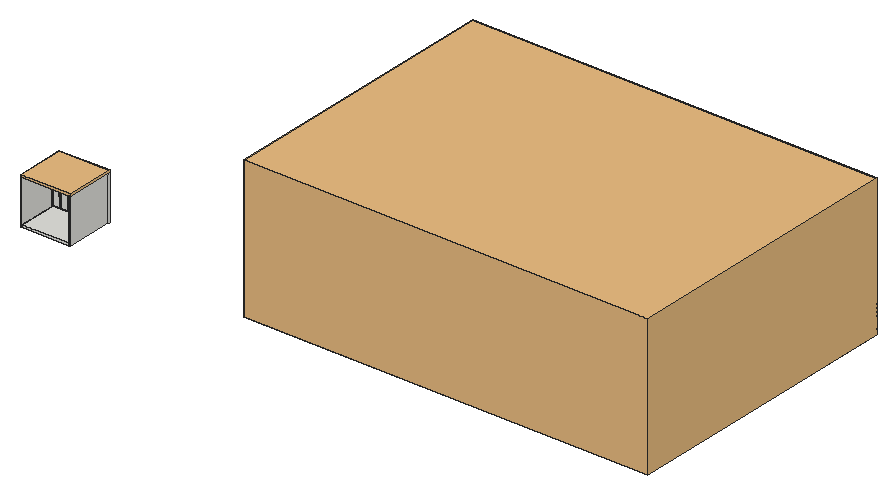
# SketchUp Ruby script. Lengths in inches.
U = 1.inch
M = Sketchup.active_model
def pt(a) = Geom::Point3d.new(a.map { |v| v * U })
def face(e, loops, mat)
  f = e.add_face(loops[0].map { |a| pt(a) })
  loops[1..].each { |l| e.add_face(l.map { |a| pt(a) }).erase! }
  f.material = f.back_material = mat if mat
  f
end
# faces: each face lists its corners as indices into pts; further lists are holes
def faces(e, pts, list, mat = nil) = list.each { |f| face(e, (f[0].is_a?(Array) ? f : [f]).map { |l| l.map { |i| pts[i] } }, mat) }
# xy, xz, yz: faces in a plane at the given z, y or x. An outline is a flat list of corners, or four numbers for a rectangle; further outlines are holes
def ring(l) = l.size == 4 ? [[l[0], l[1]], [l[2], l[1]], [l[2], l[3]], [l[0], l[3]]] : l.each_slice(2).to_a
def flat(e, list, mat, &to3) = list.each { |f| face(e, (f[0].is_a?(Array) ? f : [f]).map { |l| ring(l).map { |u, v| to3.(u, v) } }, mat) }
def xy(e, z, list, mat = nil) = flat(e, list, mat) { |x, y| [x, y, z] }
def xz(e, y, list, mat = nil) = flat(e, list, mat) { |x, z| [x, y, z] }
def yz(e, x, list, mat = nil) = flat(e, list, mat) { |y, z| [x, y, z] }
def lines(e, pts, list) = list.each { |a, b| e.add_line(pt(pts[a]), pt(pts[b])) }
# prism: a flat outline (further loops are holes) pulled along v
def prism(e, loops, v, mat = nil)
  f = face(e, loops, mat); d = Geom::Vector3d.new(v.map { |x| x * U })
  f.pushpull(f.normal.samedirection?(d) ? d.length : -d.length)
end
def box(e, o, s, mat = nil) = prism(e, [[o, [o[0] + s[0], o[1], o[2]], [o[0] + s[0], o[1] + s[1], o[2]], [o[0], o[1] + s[1], o[2]]]], [0, 0, s[2]], mat)
def at(x, y, z, deg = 0) = Geom::Transformation.translation(pt([x, y, z])) * Geom::Transformation.rotation(ORIGIN, Z_AXIS, deg.degrees)
def axes(o, x, y, z) = Geom::Transformation.new([*x, 0, *y, 0, *z, 0, *pt(o).to_a, 1])
def part(name) = M.definitions.add(name)
# library, detail: a bought-in or finely detailed component or shape, given as its bounding box
def library(name, o, s) = part(name).tap { |d| box(d.entities, o, s) }
def detail(e, o, s) = box(e.add_group.entities, o, s)
def put(e, d, t, mat = nil) = e.add_instance(d, t).tap { |i| i.material = mat if mat }
def group(e, t, mat = nil) = e.add_group.tap { |g| g.transformation = t; g.material = mat if mat }.entities
root = M.entities
M.materials.add("[Color A08]").color = [102, 0, 0]
M.materials.add("[Color M09]1").color = [0, 0, 0]
M.materials.add("[Translucent Glass Gray]1").color = [128, 128, 128]
c1 = library("Group\#158",[0,0,0],[1037.25,734.875,359.43])
c2 = part("Group299\#1")
p = [[0,0,0],[0,0,-12.87],[-0.08,0,-12.87],[0.5,-41.15,0],[-0.5,-41.15,0],[0.5,41.15,0],
  [0.5,0,0],[-0.5,41.15,0],[0.08,0,-12.87],[-0.5,0,0],[0,0,-20.82]]
lines(c2.entities,p,[[0,1],[1,2],[3,4],[5,6],[7,5],[1,8],[9,0],[0,6],[8,10],[4,9],[6,3],[2,10],
  [9,7]])
c3 = part("Rectangle Light\#5")
put(c3.entities,c2,at(0,0,0))
c4 = part("Group301\#1")
p = [[0,0,0],[0,0,-12.87],[-0.08,0,-12.87],[0.5,-41.15,0],[-0.5,-41.15,0],[0.5,41.15,0],
  [0.5,0,0],[-0.5,41.15,0],[0.08,0,-12.87],[-0.5,0,0],[0,0,-20.82]]
lines(c4.entities,p,[[0,1],[1,2],[3,4],[5,6],[7,5],[1,8],[9,0],[0,6],[8,10],[4,9],[6,3],[2,10],
  [9,7]])
c5 = part("Rectangle Light\#6")
put(c5.entities,c4,at(0,0,0))
c6 = part("Group\#164")
xy(c6.entities,0,[[1,1,2,2]])
xy(c6.entities,29.73,[[0,1,0.01,1.15,0.06,1.28,0.125,1.375,0.22,1.44,0.35,1.49,0.5,1.5,1,1.5,1,2,0,2]])
xy(c6.entities,48,[[0,1,2,1,2,2,1.15,2,1.15,1.5,0.5,1.5,0.35,1.49,0.22,1.44,0.125,1.375,0.06,1.28,0.01,1.15],[1.11,1.5,1.15,2]])
xz(c6.entities,1,[[1,0,2,0,2,48,0,48,0,29.73,0.14,29.26,0.27,28.79,0.39,28.32,0.5,27.85,0.6,27.375,0.68,26.9,0.76,26.42,0.83,25.9375,0.89,25.45,0.9375,24.97,0.97,24.49,1,24]])
xz(c6.entities,1.5,[[0.5,29.73,0.5,48,1.15,48,1.11,48,1.07,47.98,1.04,47.96,1.02,47.93,1,47.89,1,29.73]])
xz(c6.entities,2,[[1,0,1,24,0.97,24.49,0.9375,24.97,0.89,25.45,0.83,25.9375,0.76,26.42,0.68,26.9,0.6,27.375,0.5,27.85,0.39,28.32,0.27,28.79,0.14,29.26,0,29.73,1,29.73,1,47.89,1.02,47.93,1.04,47.96,1.07,47.98,1.11,48,2,48,2,0]])
yz(c6.entities,1,[[1,0,1.5,24],[1.5,0,2,24],[1.5,29.73,2,47.85],[1.5,47.85,2,47.89]])
yz(c6.entities,2,[[1,0,2,48]])
p = [[0.97,1,24.49],[0.97,1.5,24.49],[1,1.5,24],[1,1,24],[1,2,24],[0.97,2,24.49],
  [0.9375,1,24.97],[0.9375,1.5,24.97],[0.9375,2,24.97],[0.89,1,25.45],[0.89,1.5,25.45],[0.89,2,25.45],
  [0.83,1,25.9375],[0.83,1.5,25.9375],[0.83,2,25.9375],[0.76,1,26.42],[0.76,1.5,26.42],[0.76,2,26.42],
  [0.68,1,26.9],[0.68,1.5,26.9],[0.68,2,26.9],[0.6,1,27.375],[0.6,1.5,27.375],[0.6,2,27.375],
  [0.5,1,27.85],[0.5,1.5,27.85],[0.5,2,27.85],[0.39,1,28.32],[0.39,1.5,28.32],[0.39,2,28.32],
  [0.27,1,28.79],[0.27,1.5,28.79],[0.27,2,28.79],[0.14,1,29.26],[0.14,1.5,29.26],[0.14,2,29.26],
  [0,1,29.73],[0,1.5,29.73],[0,2,29.73],[0,1,48],[0.01,1.15,48],[0.01,1.15,29.73],
  [0.06,1.28,48],[0.06,1.28,29.73],[0.125,1.375,48],[0.125,1.375,29.73],[0.22,1.44,48],[0.22,1.44,29.73],
  [0.35,1.49,48],[0.35,1.49,29.73],[0.5,1.5,48],[0.5,1.5,29.73],[1,2,47.89],[1,1.5,47.89],
  [1.02,1.5,47.93],[1.02,2,47.93],[1.04,1.5,47.96],[1.04,2,47.96],[1.07,1.5,47.98],[1.07,2,47.98],
  [1.11,1.5,48],[1.11,2,48]]
faces(c6.entities,p,[[0,1,2,3],[4,2,1,5],[6,7,1,0],[5,1,7,8],[9,10,7,6],[8,7,10,11],[12,13,10,9],[11,10,13,14],
  [15,16,13,12],[14,13,16,17],[18,19,16,15],[17,16,19,20],[21,22,19,18],[20,19,22,23],[24,25,22,21],[23,22,25,26],
  [27,28,25,24],[26,25,28,29],[30,31,28,27],[29,28,31,32],[33,34,31,30],[32,31,34,35],[36,37,34,33],[35,34,37,38],
  [36,39,40,41],[41,40,42,43],[43,42,44,45],[45,44,46,47],[47,46,48,49],[49,48,50,51],[52,53,54,55],[55,54,56,57],
  [57,56,58,59],[59,58,60,61]])
c7 = part("Group\#163")
xy(c7.entities,0,[[1,1,2,2]])
xy(c7.entities,29.73,[[0,1,0.01,1.15,0.06,1.28,0.125,1.375,0.22,1.44,0.35,1.49,0.5,1.5,1,1.5,1,2,0,2]])
xy(c7.entities,48,[[0,1,2,1,2,2,1.15,2,1.15,1.5,0.5,1.5,0.35,1.49,0.22,1.44,0.125,1.375,0.06,1.28,0.01,1.15],[1.11,1.5,1.15,2]])
xz(c7.entities,1,[[1,0,2,0,2,48,0,48,0,29.73,0.14,29.26,0.27,28.79,0.39,28.32,0.5,27.85,0.6,27.375,0.68,26.9,0.76,26.42,0.83,25.9375,0.89,25.45,0.9375,24.97,0.97,24.49,1,24]])
xz(c7.entities,1.5,[[0.5,29.73,0.5,48,1.15,48,1.11,48,1.07,47.98,1.04,47.96,1.02,47.93,1,47.89,1,29.73]])
xz(c7.entities,2,[[1,0,1,24,0.97,24.49,0.9375,24.97,0.89,25.45,0.83,25.9375,0.76,26.42,0.68,26.9,0.6,27.375,0.5,27.85,0.39,28.32,0.27,28.79,0.14,29.26,0,29.73,1,29.73,1,47.89,1.02,47.93,1.04,47.96,1.07,47.98,1.11,48,2,48,2,0]])
yz(c7.entities,1,[[1,0,1.5,24],[1.5,0,2,24],[1.5,29.73,2,47.85],[1.5,47.85,2,47.89]])
yz(c7.entities,2,[[1,0,2,48]])
p = [[0.97,1,24.49],[0.97,1.5,24.49],[1,1.5,24],[1,1,24],[1,2,24],[0.97,2,24.49],
  [0.9375,1,24.97],[0.9375,1.5,24.97],[0.9375,2,24.97],[0.89,1,25.45],[0.89,1.5,25.45],[0.89,2,25.45],
  [0.83,1,25.9375],[0.83,1.5,25.9375],[0.83,2,25.9375],[0.76,1,26.42],[0.76,1.5,26.42],[0.76,2,26.42],
  [0.68,1,26.9],[0.68,1.5,26.9],[0.68,2,26.9],[0.6,1,27.375],[0.6,1.5,27.375],[0.6,2,27.375],
  [0.5,1,27.85],[0.5,1.5,27.85],[0.5,2,27.85],[0.39,1,28.32],[0.39,1.5,28.32],[0.39,2,28.32],
  [0.27,1,28.79],[0.27,1.5,28.79],[0.27,2,28.79],[0.14,1,29.26],[0.14,1.5,29.26],[0.14,2,29.26],
  [0,1,29.73],[0,1.5,29.73],[0,2,29.73],[0,1,48],[0.01,1.15,48],[0.01,1.15,29.73],
  [0.06,1.28,48],[0.06,1.28,29.73],[0.125,1.375,48],[0.125,1.375,29.73],[0.22,1.44,48],[0.22,1.44,29.73],
  [0.35,1.49,48],[0.35,1.49,29.73],[0.5,1.5,48],[0.5,1.5,29.73],[1,2,47.89],[1,1.5,47.89],
  [1.02,1.5,47.93],[1.02,2,47.93],[1.04,1.5,47.96],[1.04,2,47.96],[1.07,1.5,47.98],[1.07,2,47.98],
  [1.11,1.5,48],[1.11,2,48]]
faces(c7.entities,p,[[0,1,2,3],[4,2,1,5],[6,7,1,0],[5,1,7,8],[9,10,7,6],[8,7,10,11],[12,13,10,9],[11,10,13,14],
  [15,16,13,12],[14,13,16,17],[18,19,16,15],[17,16,19,20],[21,22,19,18],[20,19,22,23],[24,25,22,21],[23,22,25,26],
  [27,28,25,24],[26,25,28,29],[30,31,28,27],[29,28,31,32],[33,34,31,30],[32,31,34,35],[36,37,34,33],[35,34,37,38],
  [36,39,40,41],[41,40,42,43],[43,42,44,45],[45,44,46,47],[47,46,48,49],[49,48,50,51],[52,53,54,55],[55,54,56,57],
  [57,56,58,59],[59,58,60,61]])
c8 = part("Group\#165")
box(c8.entities,[0,1,-0.71],[37.13,21.125,0.71])
c9 = library("Group\#166",[0,0,0],[129,124.5,6])
put(root,c1,at(573.3125,0,-5.43))
g1 = group(root,at(4.5,0,0))
xy(g1,0,[[-4.5,0,0,120],[0,0,120,120],[120,0,124.5,120],[-4.5,120,124.5,124.5]])
xy(g1,6,[[0,0,120,120]])
xy(g1,114,[[-4.5,0,0,120],[120,0,124.5,120],[-4.5,120,124.5,124.5]])
xz(g1,0,[[-4.5,0,0,114],[0,0,120,6],[120,0,124.5,114]])
xz(g1,120,[[-4.5,0,0,6],[0,0,120,6],[120,0,124.5,6],[-4.5,6,0,114],[0,6,120,114],
  [120,6,124.5,114]])
xz(g1,124.5,[[-4.5,0,124.5,114]])
yz(g1,-4.5,[[0,0,120,114],[120,0,124.5,114]])
yz(g1,0,[[0,0,120,6],[0,6,120,114]])
yz(g1,120,[[0,0,120,6],[0,6,120,114]])
yz(g1,124.5,[[0,0,120,114],[120,0,124.5,114]])
g2 = group(root,at(4.5,96,6))
xy(g2,0,[[0,2,120,24]])
xy(g2,4,[[0,0,0,2,120,2,120,0,118,0,118,0.71,117.88,0.71,117.88,0,98.78,0,98.78,0.71,98.67,0.71,98.67,0,79.45,0,79.45,0.71,40.67,0.71,40.67,0,21.45,0,21.45,0.71,21.33,0.71,21.33,0,2.12,0,2.12,0.71,2,0.71,2,0]])
xy(g2,4,[[40.78,0,79.33,0.71]],"[Color M09]1")
xy(g2,4.71,[[41.49,1.71,42.2,1.71,42.2,2.42,77.92,2.42,77.92,1.71,78.625,1.71,78.625,22.83,41.49,22.83]])
xy(g2,4.71,[[41.49,0.71,78.625,0.71,78.625,1.71,77.92,1.71,77.92,2.42,42.2,2.42,42.2,1.71,41.49,1.71]],"[Color A08]")
xy(g2,4.71,[[41.49,0,60.12,0.24],[60.12,0,78.625,0.24],[41.49,0.24,60.06,0.71],[60.06,0.24,78.625,0.71]],"[Color M09]1")
xy(g2,4.83,[[42.32,1.71,77.8,2.42]])
xy(g2,21.88,[[42.32,1.71,57.06,2.42],[63.06,1.71,77.8,2.42]],"[Color A08]")
xy(g2,22,[[77.8,1.71,77.92,2.42]])
xy(g2,22,[[42.2,1.71,42.32,2.42],[42.32,1.71,77.8,2.42]],"[Color A08]")
xy(g2,105.72,[[41.49,0.71,78.625,22.83]],"[Color A08]")
xy(g2,105.72,[[41.49,0,60.12,0.24],[60.12,0,78.625,0.24],[41.49,0.24,60.06,0.71],[60.06,0.24,78.625,0.71]],"[Color M09]1")
xy(g2,106.31,[[2.12,0,21.33,0.71],[21.45,0,40.67,0.71],[79.45,0,98.67,0.71],[98.78,0,117.88,0.71]])
xy(g2,106.31,[[40.78,0,79.33,0.71]],"[Color M09]1")
xy(g2,106.43,[[2,0,79.33,0.71],[79.33,0,79.45,0.71],[79.45,0,118,0.71]])
xy(g2,108,[[0,0,120,24]])
xz(g2,0,[[0,4,2,4,2,106.43,118,106.43,118,4,120,4,120,108,0,108],[2.12,4,21.33,106.31],[21.45,4,40.67,106.31],[79.45,4,98.67,106.31],[98.78,4,117.88,106.31]])
xz(g2,0,[[[40.78,4,79.33,106.31],[41.49,4.71,78.625,105.72]]],"[Color M09]1")
xz(g2,0.71,[[2,4,2.12,4,2.12,106.31,21.33,106.31,21.33,4,21.45,4,21.45,106.31,40.67,106.31,40.67,4,40.78,4,40.78,106.31,79.33,106.31,79.33,106.43,2,106.43],[[40.78,4,79.33,106.31],[41.49,4.71,78.625,105.72]],[79.33,4,79.45,106.43],[98.67,4,98.78,4,98.78,106.31,117.88,106.31,117.88,4,118,4,118,106.43,79.45,106.43,79.45,106.31,98.67,106.31]])
xz(g2,1.71,[[41.49,4.71,42.2,22],[77.92,4.71,78.625,22],[42.32,4.83,77.8,4.83,77.8,21.88,63.06,21.88,62.69,21.42,62.25,21.03,61.76,20.71,61.22,20.47,60.65,20.33,60.06,20.28,59.47,20.33,58.9,20.47,58.36,20.71,57.86,21.03,57.43,21.42,57.06,21.88,42.32,21.88]],"[Color A08]")
xz(g2,2,[[0,0,120,4]])
xz(g2,2.42,[[42.32,4.71,77.8,4.83]])
xz(g2,2.42,[[42.2,4.71,42.32,22],[77.8,4.71,77.92,22],[42.32,21.88,57.06,22],[63.06,21.88,77.8,22]],"[Color A08]")
xz(g2,22.83,[[41.49,4.71,78.625,22.71],[41.49,22.71,78.625,105.72]],"[Color A08]")
xz(g2,24,[[0,0,120,108]])
yz(g2,0,[[2,0,2,4,0,4,0,108,24,108,24,0]])
yz(g2,2,[[0,4,0.71,106.43]])
yz(g2,2.12,[[0,4,0.71,106.31]])
yz(g2,21.33,[[0,4,0.71,106.31]])
yz(g2,21.45,[[0,4,0.71,106.31]])
yz(g2,40.67,[[0,4,0.71,106.31]])
yz(g2,40.78,[[0,4,0.71,106.31]],"[Color M09]1")
yz(g2,41.49,[[0.71,4.71,22.83,105.72]],"[Color A08]")
yz(g2,41.49,[[0,4.71,0.24,105.72],[0.24,4.71,0.71,105.72]],"[Color M09]1")
yz(g2,42.2,[[1.71,4.71,2.42,22]],"[Color A08]")
yz(g2,42.32,[[1.71,4.83,2.42,21.88]],"[Color A08]")
yz(g2,77.8,[[1.71,4.83,2.42,21.88]])
yz(g2,77.92,[[1.71,4.71,2.42,22]],"[Color A08]")
yz(g2,78.625,[[0.71,4.71,22.83,105.72]],"[Color A08]")
yz(g2,78.625,[[0,4.71,0.24,105.72],[0.24,4.71,0.71,105.72]],"[Color M09]1")
yz(g2,79.33,[[0,4,0.71,106.31]],"[Color M09]1")
yz(g2,79.45,[[0,4,0.71,106.31]])
yz(g2,98.67,[[0,4,0.71,106.31]])
yz(g2,98.78,[[0,4,0.71,106.31]])
yz(g2,117.88,[[0,4,0.71,106.31]])
yz(g2,118,[[0,4,0.71,106.43]])
yz(g2,120,[[2,0,24,0,24,108,0,108,0,4,2,4]])
p = [[58.9,1.71,20.47],[59.47,1.71,20.33],[59.47,2.42,20.33],[58.9,2.42,20.47],[60.06,1.71,20.28],[60.06,2.42,20.28],
  [60.65,1.71,20.33],[60.65,2.42,20.33],[61.22,1.71,20.47],[61.22,2.42,20.47],[58.36,1.71,20.71],[58.36,2.42,20.71],
  [61.76,1.71,20.71],[61.76,2.42,20.71],[57.86,1.71,21.03],[57.86,2.42,21.03],[62.25,1.71,21.03],[62.25,2.42,21.03],
  [57.43,1.71,21.42],[57.43,2.42,21.42],[62.69,1.71,21.42],[62.69,2.42,21.42],[57.06,1.71,21.88],[57.06,2.42,21.88],
  [63.06,1.71,21.88],[63.06,2.42,21.88]]
faces(g2,p,[[0,1,2,3],[1,4,5,2],[4,6,7,5],[6,8,9,7],[10,0,3,11],[8,12,13,9],[14,10,11,15],[12,16,17,13],
  [18,14,15,19],[16,20,21,17],[22,18,19,23],[20,24,25,21]],"[Color A08]")
put(g2,c3,axes([41.5,11.77,64.27],[0,1,0],[0,0,1.01],[-1,0,0]))
put(g2,c5,axes([78.61,11.77,64.21],[0,-1,0],[0,0,1.00861],[1,0,0]))
g3 = group(g2,at(23.96,-2,6),"[Color M09]1")
xy(g3,0,[[-2,1,-1,2]])
xy(g3,29.73,[[0,1,-0.01,1.15,-0.06,1.28,-0.125,1.375,-0.22,1.44,-0.35,1.49,-0.5,1.5,-1,1.5,-1,2,0,2]])
xy(g3,48,[[-2,1,-2,2,-1.15,2,-1.15,1.5,-0.5,1.5,-0.35,1.49,-0.22,1.44,-0.125,1.375,-0.06,1.28,-0.01,1.15,0,1],[-1.15,1.5,-1.11,2]])
xz(g3,1,[[-2,0,-2,48,0,48,0,29.73,-0.14,29.26,-0.27,28.79,-0.39,28.32,-0.5,27.85,-0.6,27.375,-0.68,26.9,-0.76,26.42,-0.83,25.9375,-0.89,25.45,-0.9375,24.97,-0.97,24.49,-1,24,-1,0]])
xz(g3,1.5,[[-1,29.73,-0.5,29.73,-0.5,48,-1.15,48,-1.11,48,-1.07,47.98,-1.04,47.96,-1.02,47.93,-1,47.89]])
xz(g3,2,[[-2,0,-1,0,-1,24,-0.97,24.49,-0.9375,24.97,-0.89,25.45,-0.83,25.9375,-0.76,26.42,-0.68,26.9,-0.6,27.375,-0.5,27.85,-0.39,28.32,-0.27,28.79,-0.14,29.26,0,29.73,-1,29.73,-1,47.89,-1.02,47.93,-1.04,47.96,-1.07,47.98,-1.11,48,-2,48]])
yz(g3,-2,[[1,0,2,48]])
yz(g3,-1,[[1,0,1.5,24],[1.5,0,2,24],[1.5,29.73,2,47.85],[1.5,47.85,2,47.89]])
p = [[-0.97,1,24.49],[-0.97,1.5,24.49],[-1,1.5,24],[-1,1,24],[-1,2,24],[-0.97,2,24.49],
  [-0.9375,1,24.97],[-0.9375,1.5,24.97],[-0.9375,2,24.97],[-0.89,1,25.45],[-0.89,1.5,25.45],[-0.89,2,25.45],
  [-0.83,1,25.9375],[-0.83,1.5,25.9375],[-0.83,2,25.9375],[-0.76,1,26.42],[-0.76,1.5,26.42],[-0.76,2,26.42],
  [-0.68,1,26.9],[-0.68,1.5,26.9],[-0.68,2,26.9],[-0.6,1,27.375],[-0.6,1.5,27.375],[-0.6,2,27.375],
  [-0.5,1,27.85],[-0.5,1.5,27.85],[-0.5,2,27.85],[-0.39,1,28.32],[-0.39,1.5,28.32],[-0.39,2,28.32],
  [-0.27,1,28.79],[-0.27,1.5,28.79],[-0.27,2,28.79],[-0.14,1,29.26],[-0.14,1.5,29.26],[-0.14,2,29.26],
  [0,1,29.73],[0,1.5,29.73],[0,2,29.73],[0,1,48],[-0.01,1.15,48],[-0.01,1.15,29.73],
  [-0.06,1.28,48],[-0.06,1.28,29.73],[-0.125,1.375,48],[-0.125,1.375,29.73],[-0.22,1.44,29.73],[-0.22,1.44,48],
  [-0.35,1.49,48],[-0.35,1.49,29.73],[-0.5,1.5,48],[-0.5,1.5,29.73],[-1,2,47.89],[-1,1.5,47.89],
  [-1.02,1.5,47.93],[-1.02,2,47.93],[-1.04,1.5,47.96],[-1.04,2,47.96],[-1.07,1.5,47.98],[-1.07,2,47.98],
  [-1.11,1.5,48],[-1.11,2,48]]
faces(g3,p,[[0,1,2,3],[4,2,1,5],[6,7,1,0],[5,1,7,8],[9,10,7,6],[8,7,10,11],[12,13,10,9],[11,10,13,14],
  [15,16,13,12],[14,13,16,17],[18,19,16,15],[17,16,19,20],[21,22,19,18],[20,19,22,23],[24,25,22,21],[23,22,25,26],
  [27,28,25,24],[26,25,28,29],[30,31,28,27],[29,28,31,32],[33,34,31,30],[32,31,34,35],[36,37,34,33],[35,34,37,38],
  [36,39,40,41],[41,40,42,43],[43,42,44,45],[46,47,48,49],[45,44,47,46],[49,48,50,51],[52,53,54,55],[55,54,56,57],
  [57,56,58,59],[59,58,60,61]])
put(g2,c6,axes([101.29,-2,6],[-1,0,0],[0,1,0],[0,0,1]),"[Color M09]1")
put(g2,c7,at(96.17,-2,6),"[Color M09]1")
g4 = group(g2,at(18.83,-2,6),"[Color M09]1")
xy(g4,0,[[1,1,2,2]])
xy(g4,29.73,[[0,1,0.01,1.15,0.06,1.28,0.125,1.375,0.22,1.44,0.35,1.49,0.5,1.5,1,1.5,1,2,0,2]])
xy(g4,48,[[0,1,2,1,2,2,1.15,2,1.15,1.5,0.5,1.5,0.35,1.49,0.22,1.44,0.125,1.375,0.06,1.28,0.01,1.15],[1.11,1.5,1.15,2]])
xz(g4,1,[[1,0,2,0,2,48,0,48,0,29.73,0.14,29.26,0.27,28.79,0.39,28.32,0.5,27.85,0.6,27.375,0.68,26.9,0.76,26.42,0.83,25.9375,0.89,25.45,0.9375,24.97,0.97,24.49,1,24]])
xz(g4,1.5,[[0.5,29.73,0.5,48,1.15,48,1.11,48,1.07,47.98,1.04,47.96,1.02,47.93,1,47.89,1,29.73]])
xz(g4,2,[[1,0,1,24,0.97,24.49,0.9375,24.97,0.89,25.45,0.83,25.9375,0.76,26.42,0.68,26.9,0.6,27.375,0.5,27.85,0.39,28.32,0.27,28.79,0.14,29.26,0,29.73,1,29.73,1,47.89,1.02,47.93,1.04,47.96,1.07,47.98,1.11,48,2,48,2,0]])
yz(g4,1,[[1,0,1.5,24],[1.5,0,2,24],[1.5,29.73,2,47.85],[1.5,47.85,2,47.89]])
yz(g4,2,[[1,0,2,48]])
p = [[0.97,1,24.49],[0.97,1.5,24.49],[1,1.5,24],[1,1,24],[1,2,24],[0.97,2,24.49],
  [0.9375,1,24.97],[0.9375,1.5,24.97],[0.9375,2,24.97],[0.89,1,25.45],[0.89,1.5,25.45],[0.89,2,25.45],
  [0.83,1,25.9375],[0.83,1.5,25.9375],[0.83,2,25.9375],[0.76,1,26.42],[0.76,1.5,26.42],[0.76,2,26.42],
  [0.68,1,26.9],[0.68,1.5,26.9],[0.68,2,26.9],[0.6,1,27.375],[0.6,1.5,27.375],[0.6,2,27.375],
  [0.5,1,27.85],[0.5,1.5,27.85],[0.5,2,27.85],[0.39,1,28.32],[0.39,1.5,28.32],[0.39,2,28.32],
  [0.27,1,28.79],[0.27,1.5,28.79],[0.27,2,28.79],[0.14,1,29.26],[0.14,1.5,29.26],[0.14,2,29.26],
  [0,1,29.73],[0,1.5,29.73],[0,2,29.73],[0,1,48],[0.01,1.15,48],[0.01,1.15,29.73],
  [0.06,1.28,48],[0.06,1.28,29.73],[0.125,1.375,48],[0.125,1.375,29.73],[0.22,1.44,48],[0.22,1.44,29.73],
  [0.35,1.49,48],[0.35,1.49,29.73],[0.5,1.5,48],[0.5,1.5,29.73],[1,2,47.89],[1,1.5,47.89],
  [1.02,1.5,47.93],[1.02,2,47.93],[1.04,1.5,47.96],[1.04,2,47.96],[1.07,1.5,47.98],[1.07,2,47.98],
  [1.11,1.5,48],[1.11,2,48]]
faces(g4,p,[[0,1,2,3],[4,2,1,5],[6,7,1,0],[5,1,7,8],[9,10,7,6],[8,7,10,11],[12,13,10,9],[11,10,13,14],
  [15,16,13,12],[14,13,16,17],[18,19,16,15],[17,16,19,20],[21,22,19,18],[20,19,22,23],[24,25,22,21],[23,22,25,26],
  [27,28,25,24],[26,25,28,29],[30,31,28,27],[29,28,31,32],[33,34,31,30],[32,31,34,35],[36,37,34,33],[35,34,37,38],
  [36,39,40,41],[41,40,42,43],[43,42,44,45],[45,44,46,47],[47,46,48,49],[49,48,50,51],[52,53,54,55],[55,54,56,57],
  [57,56,58,59],[59,58,60,61]])
put(g2,c8,at(41.49,0.71,22.71),"[Color A08]")
put(g2,c8,at(41.49,0.71,43.46),"[Color A08]")
put(g2,c8,at(41.49,0.71,64.21),"[Color A08]")
put(g2,c8,at(41.49,0.71,84.96),"[Color A08]")
put(g2,c6,axes([62.73,-2,6],[-1,0,0],[0,1,0],[0,0,1]),"[Color M09]1")
put(g2,c7,at(57.6,-2,6),"[Color M09]1")
g5 = group(root,at(45.99,96.125,10.71),"[Translucent Glass Gray]1")
xy(g5,0,[[17.86,-0.125,17.86,0,0,0,0,0.24,37.13,0.24,37.13,0,19.39,0,19.39,-0.125,18.68,-0.125,18.68,0,18.57,0,18.57,-0.125]])
xy(g5,101.01,[[17.86,-0.125,18.57,-0.125,18.57,0,18.68,0,18.68,-0.125,19.39,-0.125,19.39,0,37.13,0,37.13,0.24,0,0.24,0,0,17.86,0]])
xz(g5,-0.125,[[17.86,0,18.57,101.01],[18.68,0,19.39,101.01]],"[Color M09]1")
xz(g5,0,[[0,0,17.86,101.01],[19.39,0,37.13,101.01]])
yz(g5,0,[[0,0,0.24,101.01]])
yz(g5,17.86,[[-0.125,0,0,101.01]],"[Color M09]1")
yz(g5,18.57,[[-0.125,0,0,101.01]],"[Color M09]1")
yz(g5,18.68,[[-0.125,0,0,101.01]],"[Color M09]1")
yz(g5,19.39,[[-0.125,0,0,101.01]],"[Color M09]1")
yz(g5,37.13,[[0,0,0.24,101.01]])
put(root,c9,at(0,0,114))
